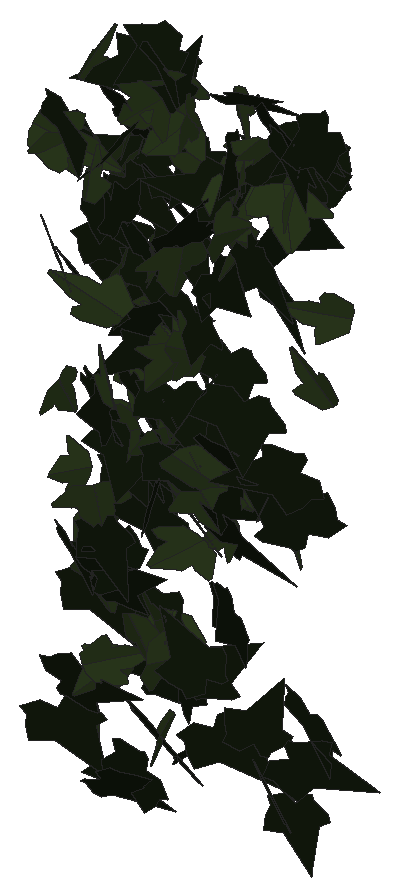
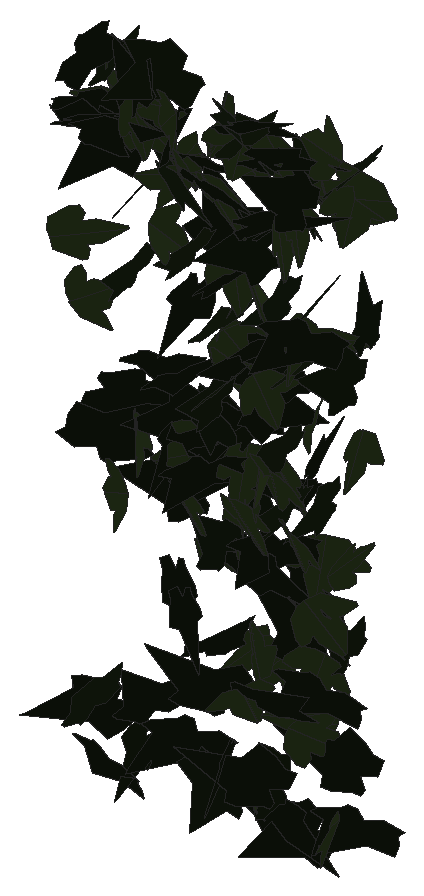
# SketchUp Ruby script. Lengths in inches.
U = 1.inch
M = Sketchup.active_model
def pt(a) = Geom::Point3d.new(a.map { |v| v * U })
def face(e, loops, mat)
  f = e.add_face(loops[0].map { |a| pt(a) })
  loops[1..].each { |l| e.add_face(l.map { |a| pt(a) }).erase! }
  f.material = f.back_material = mat if mat
  f
end
# faces: each face lists its corners as indices into pts; further lists are holes
def faces(e, pts, list, mat = nil) = list.each { |f| face(e, (f[0].is_a?(Array) ? f : [f]).map { |l| l.map { |i| pts[i] } }, mat) }
# xy, xz, yz: faces in a plane at the given z, y or x. An outline is a flat list of corners, or four numbers for a rectangle; further outlines are holes
def ring(l) = l.size == 4 ? [[l[0], l[1]], [l[2], l[1]], [l[2], l[3]], [l[0], l[3]]] : l.each_slice(2).to_a
def flat(e, list, mat, &to3) = list.each { |f| face(e, (f[0].is_a?(Array) ? f : [f]).map { |l| ring(l).map { |u, v| to3.(u, v) } }, mat) }
def xy(e, z, list, mat = nil) = flat(e, list, mat) { |x, y| [x, y, z] }
def xz(e, y, list, mat = nil) = flat(e, list, mat) { |x, z| [x, y, z] }
def yz(e, x, list, mat = nil) = flat(e, list, mat) { |y, z| [x, y, z] }
def lines(e, pts, list) = list.each { |a, b| e.add_line(pt(pts[a]), pt(pts[b])) }
# prism: a flat outline (further loops are holes) pulled along v
def prism(e, loops, v, mat = nil)
  f = face(e, loops, mat); d = Geom::Vector3d.new(v.map { |x| x * U })
  f.pushpull(f.normal.samedirection?(d) ? d.length : -d.length)
end
def box(e, o, s, mat = nil) = prism(e, [[o, [o[0] + s[0], o[1], o[2]], [o[0] + s[0], o[1] + s[1], o[2]], [o[0], o[1] + s[1], o[2]]]], [0, 0, s[2]], mat)
def at(x, y, z, deg = 0) = Geom::Transformation.translation(pt([x, y, z])) * Geom::Transformation.rotation(ORIGIN, Z_AXIS, deg.degrees)
def axes(o, x, y, z) = Geom::Transformation.new([*x, 0, *y, 0, *z, 0, *pt(o).to_a, 1])
def part(name) = M.definitions.add(name)
# library, detail: a bought-in or finely detailed component or shape, given as its bounding box
def library(name, o, s) = part(name).tap { |d| box(d.entities, o, s) }
def detail(e, o, s) = box(e.add_group.entities, o, s)
def put(e, d, t, mat = nil) = e.add_instance(d, t).tap { |i| i.material = mat if mat }
def group(e, t, mat = nil) = e.add_group.tap { |g| g.transformation = t; g.material = mat if mat }.entities
root = M.entities
M.materials.add("1026 AP 7946 SUNNY SIDE UP").color = [254, 231, 186]
M.materials.add("efeu1").color = [18, 25, 13]
M.materials.add("efeu2").color = [43, 57, 29]
c1 = part("ivyleaf_9")
p = [[1.54,2.16,1.25],[1.36,2.04,1.19],[-0.21,0.99,0.68],[-0.71,1.11,0.82],[-0.85,0.86,0.67],[-0.8,0.17,0.21],
  [-0.9,-0.01,0.1],[-0.67,-0.16,-0.02],[-0.08,-0.08,-0.05],[-0.03,-0.6,-0.4],[0.65,-0.88,-0.66],[0.83,-0.6,-0.49],
  [1.29,-0.42,-0.43],[1.8125,-0.07,-0.26],[1.21,0.44,0.15]]
faces(c1.entities,p,[[0,1,2,3,4,5,6,7,8,9,10,11,12,13,14]],"efeu1")
c2 = part("ivyleaf_10")
p = [[0,0.5,-0.03],[-0.0625,2.02,-0.43],[-0.19,2.01,-0.46],[-0.54,1.05,-0.29],[-0.52,0.625,-0.18],[-0.83,0.76,-0.28],
  [-1.16,0.64,-0.33],[-1.15,0.33,-0.24],[-0.77,-0.39,0.02],[-0.3,-0.51,0.16],[0.04,-0.48,0.23],[-0.02,2.01,-0.4375],
  [-0.06,2.01,-0.43],[0.04,-0.49,0.23],[0.67,-0.49,0.14],[1.38,0.36,-0.2],[1.375,0.51,-0.24],[0.81,0.65,-0.19],
  [0.62,0.59,-0.15],[0.6,1.09,-0.28],[0.5,1.23,-0.31]]
faces(c2.entities,p,[[0,1,2,3,4,5,6,7,8,9,10],[11,12,0,13,14,15,16,17,18,19,20]],"efeu2")
put(root,c1,axes([129.05,210.99,277.31],[-0.03614,0.17598,0.28692],[-0.11211,0.26889,-0.18017],[-0.50439,-0.07237,0.01949]),"1026 AP 7946 SUNNY SIDE UP")
put(root,c2,axes([129.63,210.99,270.41],[-0.03432,-0.08532,-0.34588],[0.18645,0.31373,-0.08837],[0.51101,-0.1202,0.00902]),"1026 AP 7946 SUNNY SIDE UP")
put(root,c2,axes([128.37,211.15,277.48],[0.34152,-0.19698,0.1294],[-0.12546,0.10026,0.30202],[-0.34626,-0.23061,0.0182]),"1026 AP 7946 SUNNY SIDE UP")
put(root,c1,axes([129.5,210.99,272.66],[0.00735,0.05181,0.32933],[0.12601,0.30928,-0.05109],[-0.49292,0.07984,-0.00815]),"1026 AP 7946 SUNNY SIDE UP")
put(root,c2,axes([129.87,211.44,275.28],[-0.13563,0.18857,0.31235],[0.17351,-0.28141,0.21175],[0.53244,0.13974,0.01056]),"1026 AP 7946 SUNNY SIDE UP")
put(root,c2,axes([127.82,211.15,274.14],[-0.03283,-0.28011,-0.17319],[0.10619,0.15953,-0.28422],[0.50128,-0.05214,0.04887]),"1026 AP 7946 SUNNY SIDE UP")
put(root,c1,axes([127.5,211.47,275.98],[-0.03711,-0.05484,0.33707],[0.04147,-0.32761,-0.05647],[0.52049,0.02219,0.02853]),"1026 AP 7946 SUNNY SIDE UP")
put(root,c1,axes([127.74,211.45,278.33],[0.03481,-0.29824,0.11718],[0.02088,-0.11476,-0.30873],[0.50242,0.02544,0.00471]),"1026 AP 7946 SUNNY SIDE UP")
put(root,c1,axes([128.38,211.4,271.9],[-0.18899,-0.07926,-0.29691],[0.45995,0.0304,-0.13431],[0.09331,-0.31036,0.06072]),"1026 AP 7946 SUNNY SIDE UP")
put(root,c1,axes([128.37,211.53,273.72],[-0.04724,-0.04377,0.32393],[-0.18006,-0.29336,-0.05502],[0.466,-0.11779,0.01158]),"1026 AP 7946 SUNNY SIDE UP")
put(root,c1,axes([127.77,211.33,269.29],[0.15816,-0.02647,0.30557],[0.40037,-0.15502,-0.10406],[0.24328,0.27232,-0.02741]),"1026 AP 7946 SUNNY SIDE UP")
put(root,c1,axes([130.28,211.3,270.26],[-0.3211,-0.23771,0.08691],[0.07017,0.07455,0.32295],[-0.39109,0.20854,-0.01341]),"1026 AP 7946 SUNNY SIDE UP")
put(root,c1,axes([128.62,211.16,268.06],[0.40552,0.09724,0.12037],[0.18187,0.0221,-0.28317],[-0.15406,0.28204,-0.01745]),"1026 AP 7946 SUNNY SIDE UP")
put(root,c2,axes([129.04,211.37,270.59],[-0.35639,0.14158,-0.17829],[0.18327,-0.13681,-0.27208],[-0.30119,-0.25077,0.04541]),"1026 AP 7946 SUNNY SIDE UP")
put(root,c1,axes([130.42,211.39,272.68],[0.39243,-0.15198,0.2279],[0.26686,-0.14617,-0.30039],[0.32839,0.3004,-0.02824]),"1026 AP 7946 SUNNY SIDE UP")
put(root,c2,axes([130.33,211.29,273.13],[-0.40898,-0.16433,-0.12112],[0.1824,0.03363,-0.3151],[0.2591,-0.28306,0.03064]),"1026 AP 7946 SUNNY SIDE UP")
put(root,c2,axes([128.52,211.36,275.53],[0.20612,0.11642,0.29651],[-0.42789,-0.10587,0.17157],[0.23302,-0.29738,0.05277]),"1026 AP 7946 SUNNY SIDE UP")
put(root,c2,axes([129.72,211.46,275.13],[-0.25431,-0.23326,0.17969],[-0.13068,-0.15583,-0.29277],[0.44024,-0.181,0.01689]),"1026 AP 7946 SUNNY SIDE UP")
put(root,c2,axes([128.48,211.57,269.72],[-0.1363,-0.14764,0.29177],[-0.05804,-0.28771,-0.16735],[0.50003,-0.07364,0.0601]),"1026 AP 7946 SUNNY SIDE UP")
put(root,c1,axes([128.74,211.375,278.28],[-0.25616,0.23861,-0.13454],[0.10278,-0.11505,-0.29814],[-0.41623,-0.17526,0.00918]),"1026 AP 7946 SUNNY SIDE UP")
put(root,c2,axes([128.28,211.36,272.48],[-0.34105,-0.26769,-0.06622],[0.09035,0.03403,-0.35395],[0.42278,-0.22322,0.02223]),"1026 AP 7946 SUNNY SIDE UP")
put(root,c1,axes([129.14,211.37,268.3],[0.00321,-0.00182,-0.33244],[-0.48191,-0.10101,-0.002],[-0.15881,0.30647,-0.00064]),"1026 AP 7946 SUNNY SIDE UP")
put(root,c2,axes([127.52,211.31,278],[0.14965,0.07463,0.37441],[0.5105,0.16395,-0.12145],[-0.28102,0.33757,-0.02126]),"1026 AP 7946 SUNNY SIDE UP")
put(root,c1,axes([129.54,211.67,273.75],[0.02842,-0.14495,0.33949],[0.10059,-0.32425,-0.15206],[0.55827,0.0658,0.01011]),"1026 AP 7946 SUNNY SIDE UP")
put(root,c1,axes([128.26,211.45,271.1],[0.48389,-0.00134,-0.17581],[0.25625,0.10678,0.30251],[0.07967,-0.3353,0.09488]),"1026 AP 7946 SUNNY SIDE UP")
put(root,c2,axes([128.59,211.27,274.2],[-0.11055,0.24722,-0.18281],[-0.09003,0.16959,0.26568],[0.47127,0.09039,0.00787]),"1026 AP 7946 SUNNY SIDE UP")
put(root,c1,axes([131.02,211.41,277.27],[0.2482,-0.26604,-0.16115],[-0.12632,0.13247,-0.31791],[0.46731,0.17711,-0.00035]),"1026 AP 7946 SUNNY SIDE UP")
put(root,c2,axes([127.73,211.41,277.95],[-0.30314,-0.24559,-0.07311],[0.10429,0.036,-0.32003],[0.38759,-0.20177,0.02893]),"1026 AP 7946 SUNNY SIDE UP")
put(root,c2,axes([130.63,211.2,277.56],[-0.02095,-0.10662,-0.33952],[0.12533,0.31939,-0.1081],[0.52911,-0.07988,0.01216]),"1026 AP 7946 SUNNY SIDE UP")
put(root,c1,axes([128.76,211.59,273.38],[-0.27246,-0.23955,-0.03389],[0.04668,0.01741,-0.30414],[0.37704,-0.17526,0.01317]),"1026 AP 7946 SUNNY SIDE UP")
put(root,c1,axes([131.66,211.66,273.84],[-0.0955,-0.10077,-0.31666],[-0.13134,-0.29666,0.11567],[-0.4905,0.09906,0.03068]),"1026 AP 7946 SUNNY SIDE UP")
put(root,c1,axes([127.64,211.66,271.25],[0.0968,-0.20808,0.21064],[0.0783,-0.19963,-0.22462],[0.45331,0.07892,-0.00618]),"1026 AP 7946 SUNNY SIDE UP")
put(root,c1,axes([127.57,211.45,268.68],[-0.13261,-0.14281,-0.27571],[0.24065,0.21883,-0.16922],[0.41053,-0.17441,0.01014]),"1026 AP 7946 SUNNY SIDE UP")
put(root,c1,axes([130.74,211.3,273.38],[0.07161,-0.09106,-0.32178],[-0.28611,0.2537,-0.10221],[0.42315,0.18695,-0.01465]),"1026 AP 7946 SUNNY SIDE UP")
put(root,c1,axes([128.83,211.32,271.45],[-0.22133,0.23155,0.22346],[-0.2025,0.1736,-0.27769],[-0.4544,-0.19015,0.01491]),"1026 AP 7946 SUNNY SIDE UP")
put(root,c2,axes([128.41,211.28,269.8125],[-0.06367,-0.07271,0.31966],[0.1641,0.29295,0.08635],[-0.47416,0.11115,-0.01304]),"1026 AP 7946 SUNNY SIDE UP")
put(root,c2,axes([129.92,211.44,273.47],[-0.35848,-0.04406,-0.32485],[0.49807,0.00473,-0.23677],[0.04667,-0.38888,0.03162]),"1026 AP 7946 SUNNY SIDE UP")
put(root,c2,axes([131.55,211.69,278.46],[0.24892,-0.15151,0.277],[0.24832,-0.22098,-0.22465],[0.41831,0.22133,-0.03148]),"1026 AP 7946 SUNNY SIDE UP")
put(root,c1,axes([130.22,211.48,273.78],[0.43052,-0.08553,0.13979],[0.19363,-0.06142,-0.29517],[0.16263,0.29957,-0.01863]),"1026 AP 7946 SUNNY SIDE UP")
put(root,c1,axes([130.71,211.64,274.62],[-0.28987,-0.25054,-0.11803],[0.15156,0.06868,-0.31804],[0.40483,-0.20511,0.03456]),"1026 AP 7946 SUNNY SIDE UP")
put(root,c2,axes([127.72,211.73,272.51],[-0.09263,0.0901,0.31063],[0.0734,-0.30035,0.10027],[0.48859,0.06221,0.04383]),"1026 AP 7946 SUNNY SIDE UP")
put(root,c1,axes([129.61,211.52,273.5],[-0.12331,-0.18731,-0.22803],[0.18354,0.18831,-0.20666],[0.41597,-0.13861,0.02359]),"1026 AP 7946 SUNNY SIDE UP")
put(root,c2,axes([129.84,211.58,272.08],[0.38296,-0.01189,-0.19114],[-0.29222,-0.01848,-0.25029],[-0.00277,0.30557,-0.02078]),"1026 AP 7946 SUNNY SIDE UP")
put(root,c1,axes([131.82,211.65,272.97],[0.12164,0.0534,0.35362],[-0.53828,-0.04622,0.08669],[0.09002,-0.34852,0.04056]),"1026 AP 7946 SUNNY SIDE UP")
put(root,c2,axes([129.09,211.68,270.56],[-0.26199,0.11489,0.2469],[0.30605,-0.13875,0.20767],[0.28322,0.2562,0.00398]),"1026 AP 7946 SUNNY SIDE UP")
put(root,c1,axes([131.45,211.78,278.87],[0.07747,-0.27477,0.16978],[0.04162,-0.16427,-0.28853],[0.50335,0.05587,-0.00227]),"1026 AP 7946 SUNNY SIDE UP")
put(root,c2,axes([131.47,211.6,278.22],[0.4872,0.15852,0.05341],[0.09277,-0.00388,-0.35723],[-0.24483,0.31398,-0.02907]),"1026 AP 7946 SUNNY SIDE UP")
put(root,c1,axes([130.68,211.46,271.32],[0.21084,-0.05168,-0.36213],[-0.54662,0.05702,-0.14503],[0.1132,0.3716,-0.02584]),"1026 AP 7946 SUNNY SIDE UP")
put(root,c2,axes([130.53,211.55,272.61],[0.26905,-0.19486,-0.17393],[-0.19767,0.11233,-0.26592],[0.35264,0.21164,-0.01636]),"1026 AP 7946 SUNNY SIDE UP")
put(root,c1,axes([129.5625,211.63,276.83],[0.3047,0.25585,0.16376],[-0.17667,-0.11212,0.32937],[0.43815,-0.22313,0.01892]),"1026 AP 7946 SUNNY SIDE UP")
put(root,c1,axes([128.83,211.7,268.92],[0.39636,-0.20678,0.09989],[0.09417,-0.08132,-0.33546],[0.34737,0.25799,-0.02304]),"1026 AP 7946 SUNNY SIDE UP")
put(root,c1,axes([131.125,211.58,268.75],[0.36382,-0.11912,-0.19706],[-0.27812,0.07231,-0.26731],[0.21808,0.29093,-0.01215]),"1026 AP 7946 SUNNY SIDE UP")
put(root,c1,axes([130.32,211.73,277.79],[-0.33953,0.10209,0.19611],[-0.33432,-0.05712,-0.21789],[-0.05525,-0.28175,0.1133]),"1026 AP 7946 SUNNY SIDE UP")
put(root,c1,axes([129.43,211.73,274.31],[-0.18884,-0.23136,-0.19199],[0.20956,0.13614,-0.26366],[0.41605,-0.17359,0.04566]),"1026 AP 7946 SUNNY SIDE UP")
put(root,c1,axes([129.63,211.91,275.59],[-0.07289,-0.26866,0.17676],[0.0389,-0.17741,-0.27786],[0.50103,-0.02531,0.04729]),"1026 AP 7946 SUNNY SIDE UP")
put(root,c2,axes([129.54,211.69,276.6],[-0.22282,-0.35213,-0.00676],[0.01818,0.00027,-0.39088],[0.55344,-0.14178,0.01012]),"1026 AP 7946 SUNNY SIDE UP")
put(root,c1,axes([131.54,211.8,268.38],[-0.23612,-0.10876,-0.25877],[0.4151,0.01566,-0.1699],[0.11032,-0.2917,0.08541]),"1026 AP 7946 SUNNY SIDE UP")
put(root,c2,axes([128.75,211.59,273.5625],[0.18675,-0.1689,-0.22156],[-0.20642,0.16929,-0.2116],[0.37586,0.17689,-0.00612]),"1026 AP 7946 SUNNY SIDE UP")
put(root,c2,axes([129.22,211.8,268.9],[0.18981,-0.2778,0.08354],[0.04155,-0.07863,-0.31242],[0.45385,0.12338,-0.00634]),"1026 AP 7946 SUNNY SIDE UP")
put(root,c1,axes([129.75,211.81,273.33],[-0.12644,-0.28418,-0.12347],[0.09737,0.10477,-0.30219],[0.47409,-0.09731,0.02913]),"1026 AP 7946 SUNNY SIDE UP")
put(root,c2,axes([128.09,211.71,270.99],[-0.45802,0.04273,-0.03487],[0.04652,-0.03222,-0.30216],[-0.07229,-0.2915,0.02653]),"1026 AP 7946 SUNNY SIDE UP")
put(root,c2,axes([129.3,211.7,273.64],[-0.21056,-0.31844,-0.1078],[0.09808,0.08506,-0.35455],[0.51695,-0.14584,0.02336]),"1026 AP 7946 SUNNY SIDE UP")
put(root,c2,axes([131.2,211.62,273.45],[0.06736,-0.22943,-0.23593],[-0.05886,0.22464,-0.2391],[0.50486,0.0568,0.0036]),"1026 AP 7946 SUNNY SIDE UP")
put(root,c1,axes([130.92,211.64,269.3],[-0.21703,-0.07994,0.28471],[0.35832,0.15755,0.16484],[-0.27725,0.26619,-0.00982]),"1026 AP 7946 SUNNY SIDE UP")
put(root,c1,axes([129.47,211.97,272.33],[0.11596,-0.19536,0.23884],[0.1538,-0.21171,-0.21605],[0.45263,0.12199,0.01223]),"1026 AP 7946 SUNNY SIDE UP")
put(root,c1,axes([130.2,211.68,269.1875],[-0.0315,-0.1298,-0.32335],[0.13825,0.30095,-0.13255],[0.51475,-0.08877,0.01582]),"1026 AP 7946 SUNNY SIDE UP")
put(root,c1,axes([129.73,211.68,269.88],[-0.14882,0.04494,0.33821],[0.51858,-0.01741,0.10038],[0.04609,0.34098,-0.03742]),"1026 AP 7946 SUNNY SIDE UP")
put(root,c1,axes([128.46,211.97,274.12],[0.17967,-0.26996,0.11947],[0.04261,-0.11586,-0.30206],[0.46098,0.11593,-0.01864]),"1026 AP 7946 SUNNY SIDE UP")
put(root,c1,axes([128.77,212.02,274.77],[-0.04971,-0.0176,-0.31547],[0.08135,-0.30364,0.0107],[-0.47523,-0.05013,0.03483]),"1026 AP 7946 SUNNY SIDE UP")
put(root,c1,axes([130.28,212.09,278.31],[0.0741,-0.13063,-0.33134],[0.37427,-0.2231,0.12827],[-0.39584,-0.2354,0.05926]),"1026 AP 7946 SUNNY SIDE UP")
put(root,c1,axes([128.57,211.75,277.42],[0.19747,-0.22015,-0.21757],[-0.03881,0.219,-0.25052],[0.47676,0.10902,0.06972]),"1026 AP 7946 SUNNY SIDE UP")
put(root,c1,axes([131.59,211.66,269.2],[0.12632,-0.00609,-0.33161],[0.13688,0.31978,0.01803],[0.48732,-0.08824,0.0809]),"1026 AP 7946 SUNNY SIDE UP")
put(root,c1,axes([127.875,211.87,270.73],[-0.15224,-0.14506,-0.29215],[0.36536,0.16936,-0.17047],[0.34092,-0.24627,0.05223]),"1026 AP 7946 SUNNY SIDE UP")
put(root,c1,axes([128.38,211.98,273.3],[0.21304,-0.30874,0.04991],[0.01434,-0.05079,-0.34742],[0.49163,0.13527,-0.0115]),"1026 AP 7946 SUNNY SIDE UP")
put(root,c1,axes([127.375,211.95,275.53],[0.30523,-0.20718,0.13057],[0.10652,-0.11119,-0.29207],[0.36775,0.20417,-0.02378]),"1026 AP 7946 SUNNY SIDE UP")
put(root,c2,axes([129.42,211.74,272.91],[-0.30461,0.20774,0.15184],[-0.19543,0.08285,-0.29044],[-0.34836,-0.22813,0.03017]),"1026 AP 7946 SUNNY SIDE UP")
put(root,c1,axes([130.34,211.74,271.15],[0.16429,-0.00982,-0.29922],[-0.45078,0.04681,-0.10761],[0.07446,0.30505,0.00871]),"1026 AP 7946 SUNNY SIDE UP")
put(root,c1,axes([129.21,211.87,272.26],[-0.10269,-0.06167,-0.34231],[-0.4897,-0.11951,0.0853],[-0.20494,0.31648,-0.0323]),"1026 AP 7946 SUNNY SIDE UP")
put(root,c2,axes([129.64,211.73,278.83],[0.10451,-0.24989,-0.2202],[0.07877,0.22184,-0.25152],[0.50956,0.01696,0.08404]),"1026 AP 7946 SUNNY SIDE UP")
put(root,c2,axes([127.9375,212.01,271.93],[-0.18647,-0.26357,0.17374],[-0.0561,-0.16938,-0.29692],[0.49008,-0.11967,0.03212]),"1026 AP 7946 SUNNY SIDE UP")
put(root,c1,axes([128.22,212.13,275.48],[-0.09831,-0.24482,0.20275],[0.00266,-0.20233,-0.25809],[0.49529,-0.04751,0.04163]),"1026 AP 7946 SUNNY SIDE UP")
put(root,c1,axes([131.51,211.63,277.78],[-0.02008,-0.01392,-0.38079],[-0.16128,0.3554,-0.00806],[0.55868,0.1021,-0.01602]),"1026 AP 7946 SUNNY SIDE UP")
put(root,c2,axes([132.01,211.81,275.16],[-0.30346,0.08546,-0.23411],[-0.30022,0.12689,0.21648],[0.23697,0.2702,-0.02553]),"1026 AP 7946 SUNNY SIDE UP")
put(root,c2,axes([130.23,212.04,278.09],[0.35073,-0.19127,0.1937],[0.20538,-0.13774,-0.30303],[0.36972,0.25796,-0.01541]),"1026 AP 7946 SUNNY SIDE UP")
put(root,c1,axes([131.74,212.18,279.09],[0.00092,-0.09785,-0.3563],[0.21978,-0.31797,0.09122],[-0.51977,-0.13463,0.03794]),"1026 AP 7946 SUNNY SIDE UP")
put(root,c1,axes([129.77,212.02,274.39],[-0.25176,0.14709,-0.24337],[0.23016,-0.18842,-0.22337],[-0.37347,-0.21527,0.0264]),"1026 AP 7946 SUNNY SIDE UP")
put(root,c2,axes([128.98,211.91,276.3125],[0.19381,-0.29904,-0.12059],[-0.08626,0.10209,-0.33241],[0.49654,0.13446,-0.01068]),"1026 AP 7946 SUNNY SIDE UP")
put(root,c2,axes([129.31,211.99,278.44],[0.42918,-0.0202,-0.15071],[-0.23129,-0.01263,-0.28122],[0.01858,0.30937,-0.0195]),"1026 AP 7946 SUNNY SIDE UP")
put(root,c1,axes([128.71,211.71,275.26],[0.03175,0.15851,-0.28587],[0.06495,0.27532,0.1662],[0.49952,-0.04587,-0.00344]),"1026 AP 7946 SUNNY SIDE UP")
put(root,c2,axes([130.33,211.68,277.54],[0.19639,0.05672,-0.36876],[0.25659,0.32962,0.1143],[0.50939,-0.1879,0.0846]),"1026 AP 7946 SUNNY SIDE UP")
put(root,c1,axes([128.4,212.02,276.45],[0.29956,-0.24546,-0.00482],[-0.02119,-0.0063,-0.31978],[0.38541,0.19043,-0.01383]),"1026 AP 7946 SUNNY SIDE UP")
put(root,c2,axes([129.32,211.92,274.94],[0.33559,0.0338,0.23023],[-0.35411,0.00902,0.22041],[0.02639,-0.30875,0.02981]),"1026 AP 7946 SUNNY SIDE UP")
put(root,c2,axes([128.33,211.88,275.9],[0.00432,-0.26828,-0.16607],[0.04458,0.15924,-0.27418],[0.48888,-0.01215,0.02647]),"1026 AP 7946 SUNNY SIDE UP")
put(root,c1,axes([131.15,212.11,278.32],[-0.39124,-0.17673,-0.13588],[0.20572,0.03992,-0.3115],[0.27797,-0.2783,0.03928]),"1026 AP 7946 SUNNY SIDE UP")
put(root,c2,axes([128.27,211.96,277.77],[0.00856,-0.31122,-0.06673],[0.01866,0.06318,-0.32003],[0.49894,0.00298,0.01311]),"1026 AP 7946 SUNNY SIDE UP")
put(root,c2,axes([132.01,212.14,276.27],[-0.04892,-0.04845,-0.31888],[-0.41692,-0.16111,0.05254],[-0.26163,0.2658,-0.0241]),"1026 AP 7946 SUNNY SIDE UP")
put(root,c2,axes([130.37,212.1875,276.91],[0.06662,-0.23372,0.22661],[0.03384,-0.22065,-0.2456],[0.50497,0.04562,-0.01344]),"1026 AP 7946 SUNNY SIDE UP")
put(root,c2,axes([128.8125,211.95,278.66],[0.39616,-0.11657,-0.19844],[-0.24741,0.11423,-0.28354],[0.25197,0.29543,0.03359]),"1026 AP 7946 SUNNY SIDE UP")
put(root,c2,axes([129.08,212.07,270.36],[0.25776,0.24129,-0.12512],[-0.07733,-0.11466,-0.30034],[-0.41865,0.16974,-0.02156]),"1026 AP 7946 SUNNY SIDE UP")
put(root,c2,axes([131.08,212.16,272.71],[-0.16714,0.17126,-0.29552],[0.19771,-0.25948,-0.20841],[-0.48812,-0.16375,0.01677]),"1026 AP 7946 SUNNY SIDE UP")
put(root,c2,axes([127.67,211.96,268.77],[-0.13051,0.29732,0.00455],[-0.01614,-0.00003,-0.31784],[-0.46725,-0.08304,0.00971]),"1026 AP 7946 SUNNY SIDE UP")
put(root,c2,axes([130.68,212.16,278.4375],[-0.22846,-0.2091,0.18078],[-0.0577,-0.18333,-0.2557],[0.42655,-0.13679,0.06224]),"1026 AP 7946 SUNNY SIDE UP")
put(root,c1,axes([128.53,212.01,272.79],[-0.08996,-0.23833,-0.24565],[0.08583,0.23073,-0.25115],[0.5216,-0.07907,-0.00104]),"1026 AP 7946 SUNNY SIDE UP")
put(root,c1,axes([130.74,212.22,278.78],[0.00322,-0.06148,0.32102],[0.14858,-0.29775,-0.06283],[0.47737,0.09309,0.01739]),"1026 AP 7946 SUNNY SIDE UP")
put(root,c1,axes([129.71,211.78,268.72],[0.13243,0.26424,0.16428],[0.09356,0.14671,-0.28464],[-0.47494,0.10258,-0.01027]),"1026 AP 7946 SUNNY SIDE UP")
put(root,c1,axes([127.81,211.94,276.75],[0.27363,-0.18321,-0.21063],[-0.17395,0.17342,-0.25739],[0.39375,0.20393,0.03267]),"1026 AP 7946 SUNNY SIDE UP")
put(root,c2,axes([129.61,212.03,277.76],[0.36681,-0.17158,-0.15404],[-0.19742,0.07989,-0.29771],[0.29727,0.26477,-0.00764]),"1026 AP 7946 SUNNY SIDE UP")
put(root,c1,axes([129.22,212.14,276.63],[0.05548,-0.31802,-0.06577],[0.00959,0.06304,-0.329],[0.5094,0.03345,0.01336]),"1026 AP 7946 SUNNY SIDE UP")
put(root,c1,axes([128.8,212.22,277.53],[-0.20215,-0.26084,-0.19052],[-0.15465,-0.15573,0.2982],[-0.47699,0.16104,-0.01594]),"1026 AP 7946 SUNNY SIDE UP")
put(root,c1,axes([127.64,212.06,273.71],[0.33979,-0.21037,-0.08917],[-0.11159,0.04935,-0.31008],[0.33909,0.22704,-0.01269]),"1026 AP 7946 SUNNY SIDE UP")
put(root,c1,axes([130.03,212.22,274.9],[-0.09374,-0.31287,-0.02687],[0.01537,0.02288,-0.32794],[0.49321,-0.06018,0.00511]),"1026 AP 7946 SUNNY SIDE UP")
put(root,c1,axes([130.32,212.17,277.87],[-0.37421,0.15225,-0.16292],[0.18706,-0.10809,-0.29067],[-0.29126,-0.26503,0.02264]),"1026 AP 7946 SUNNY SIDE UP")
put(root,c2,axes([127.71,211.95,278.85],[0.09868,-0.24542,0.22966],[-0.07534,0.21922,0.26217],[-0.51735,-0.07873,0.00562]),"1026 AP 7946 SUNNY SIDE UP")
put(root,c1,axes([128.84,212.04,270.31],[-0.47907,-0.07031,-0.06274],[-0.10234,0.01405,0.32092],[-0.10391,0.3103,-0.02684]),"1026 AP 7946 SUNNY SIDE UP")
put(root,c1,axes([128.57,212.22,275.91],[0.01277,-0.30356,-0.06353],[0.01431,0.06017,-0.3123],[0.48633,0.0062,0.01086]),"1026 AP 7946 SUNNY SIDE UP")
put(root,c1,axes([131.35,212.36,269.52],[0.06279,-0.29172,0.21636],[0.09039,-0.20509,-0.30355],[0.55948,0.06588,0.02476]),"1026 AP 7946 SUNNY SIDE UP")
put(root,c1,axes([127.96,212.28,278.13],[0.23917,-0.14898,0.24409],[0.22518,-0.19137,-0.21902],[0.37942,0.20749,-0.02388]),"1026 AP 7946 SUNNY SIDE UP")
put(root,c1,axes([130.25,211.97,279.26],[0.44414,0.08661,0.10557],[0.11468,0.10006,-0.29505],[-0.17638,0.28315,0.07399]),"1026 AP 7946 SUNNY SIDE UP")
put(root,c2,axes([128.375,212.15,277.59],[0.03593,-0.31143,-0.06234],[0.0264,0.06001,-0.32063],[0.49763,0.0193,0.02151]),"1026 AP 7946 SUNNY SIDE UP")
put(root,c2,axes([130.76,212.19,278.58],[-0.10956,-0.31002,0.00465],[0.01254,-0.00822,-0.32725],[0.48741,-0.06948,0.00946]),"1026 AP 7946 SUNNY SIDE UP")
put(root,c1,axes([129.55,212.3,277.95],[-0.45957,-0.03879,-0.11087],[0.17567,-0.03608,-0.29999],[0.03715,-0.30928,0.04704]),"1026 AP 7946 SUNNY SIDE UP")
put(root,c1,axes([128.63,212.2,277.26],[0.44234,-0.15905,0.08392],[0.08482,-0.071,-0.33147],[0.26856,0.2844,-0.03353]),"1026 AP 7946 SUNNY SIDE UP")
put(root,c2,axes([128.63,212.28,275.21],[-0.16457,-0.27543,0.10246],[0.00819,-0.10898,-0.3012],[0.46123,-0.09634,0.0419]),"1026 AP 7946 SUNNY SIDE UP")
put(root,c2,axes([128.56,212.41,273.55],[-0.13218,0.06783,0.3034],[0.27976,-0.2355,0.10696],[0.3834,0.19522,0.02655]),"1026 AP 7946 SUNNY SIDE UP")
put(root,c1,axes([130.67,212.34,276.24],[0.19949,-0.28429,0.05617],[0.01412,-0.0574,-0.32068],[0.45544,0.12631,-0.01466]),"1026 AP 7946 SUNNY SIDE UP")
put(root,c1,axes([129.56,212.21,273.67],[-0.00831,-0.26766,-0.22901],[0.01652,0.22057,-0.27446],[0.54531,-0.01076,0.00483]),"1026 AP 7946 SUNNY SIDE UP")
put(root,c1,axes([127.89,212.17,276.2],[-0.07298,-0.13024,-0.29842],[0.15927,0.2706,-0.14084],[0.4722,-0.1114,0.00139]),"1026 AP 7946 SUNNY SIDE UP")
put(root,c1,axes([129.84,212.09,276.18],[0.07177,-0.13379,-0.32845],[-0.24956,0.27674,-0.14177],[0.48177,0.16328,-0.02451]),"1026 AP 7946 SUNNY SIDE UP")
put(root,c1,axes([131.58,212.47,278.27],[-0.36395,-0.08649,0.1858],[-0.18377,-0.16621,-0.23696],[0.25609,-0.24218,0.09401]),"1026 AP 7946 SUNNY SIDE UP")
put(root,c2,axes([128.31,212.37,274],[0.43747,-0.11705,0.10198],[0.12157,-0.07156,-0.30937],[0.20892,0.28673,-0.03352]),"1026 AP 7946 SUNNY SIDE UP")
put(root,c1,axes([128.97,212.07,278.71],[-0.33493,0.28216,-0.03268],[-0.0072,0.03823,0.36389],[0.4467,0.21218,-0.01863]),"1026 AP 7946 SUNNY SIDE UP")
put(root,c2,axes([127.96,212.38,273.2],[0.37224,-0.15047,0.0795],[0.08184,-0.06302,-0.28825],[0.25364,0.24116,-0.02366]),"1026 AP 7946 SUNNY SIDE UP")
put(root,c1,axes([129.09,212.45,275.15],[0.08194,-0.32268,0.04257],[0.00113,-0.04359,-0.33693],[0.5119,0.05175,-0.00607]),"1026 AP 7946 SUNNY SIDE UP")
put(root,c2,axes([128.94,212.34,273.29],[0.38399,-0.14753,-0.08693],[-0.13386,0.01999,-0.2926],[0.23054,0.25733,-0.0251]),"1026 AP 7946 SUNNY SIDE UP")
put(root,c1,axes([129.25,212.16,269.45],[0.15289,-0.06401,-0.29363],[-0.33143,0.19205,-0.11754],[0.31721,0.23152,0.01871]),"1026 AP 7946 SUNNY SIDE UP")
put(root,c1,axes([128.46,212.51,278.79],[-0.36906,-0.05296,0.22018],[-0.29775,-0.1117,-0.24306],[0.17758,-0.29735,0.05005]),"1026 AP 7946 SUNNY SIDE UP")
put(root,c1,axes([128.66,212.57,278.99],[-0.0354,-0.24417,0.20204],[0.08791,-0.19796,-0.24672],[0.48592,0.01802,0.05935]),"1026 AP 7946 SUNNY SIDE UP")
put(root,c1,axes([129.18,212.45,274.88],[0.26865,-0.24991,0.06735],[0.02873,-0.06819,-0.31138],[0.40574,0.1703,-0.02254]),"1026 AP 7946 SUNNY SIDE UP")
put(root,c1,axes([128.56,212.26,269.21],[0.09277,0.02281,0.31959],[0.48695,-0.03259,-0.05842],[0.04381,0.31397,-0.02742]),"1026 AP 7946 SUNNY SIDE UP")
put(root,c2,axes([128.87,212.34,278.9],[-0.47757,-0.04216,-0.03415],[0.05847,-0.03004,-0.31404],[0.06045,-0.30402,0.03394]),"1026 AP 7946 SUNNY SIDE UP")
put(root,c1,axes([131.51,212.35,278.11],[-0.09238,0.05868,0.32198],[-0.46723,0.10215,-0.07679],[-0.17668,-0.30082,0.03471]),"1026 AP 7946 SUNNY SIDE UP")
put(root,c1,axes([131.44,212.55,278.69],[-0.31189,-0.22328,0.06389],[-0.04636,-0.05834,-0.30756],[0.36196,-0.19987,0.01567]),"1026 AP 7946 SUNNY SIDE UP")
put(root,c1,axes([128.76,212.58,279.21],[-0.39304,-0.14636,0.12216],[-0.10418,-0.11755,-0.29199],[0.27815,-0.25085,0.06326]),"1026 AP 7946 SUNNY SIDE UP")
put(root,c1,axes([129.59,212.47,276.97],[0.20401,-0.27973,0.02653],[0.02144,-0.02381,-0.3178],[0.44143,0.13044,0.00318]),"1026 AP 7946 SUNNY SIDE UP")
put(root,c2,axes([129.99,212.48,278.91],[-0.23581,0.17392,-0.21252],[0.11558,-0.20189,-0.23048],[-0.40946,-0.15715,0.05733]),"1026 AP 7946 SUNNY SIDE UP")
